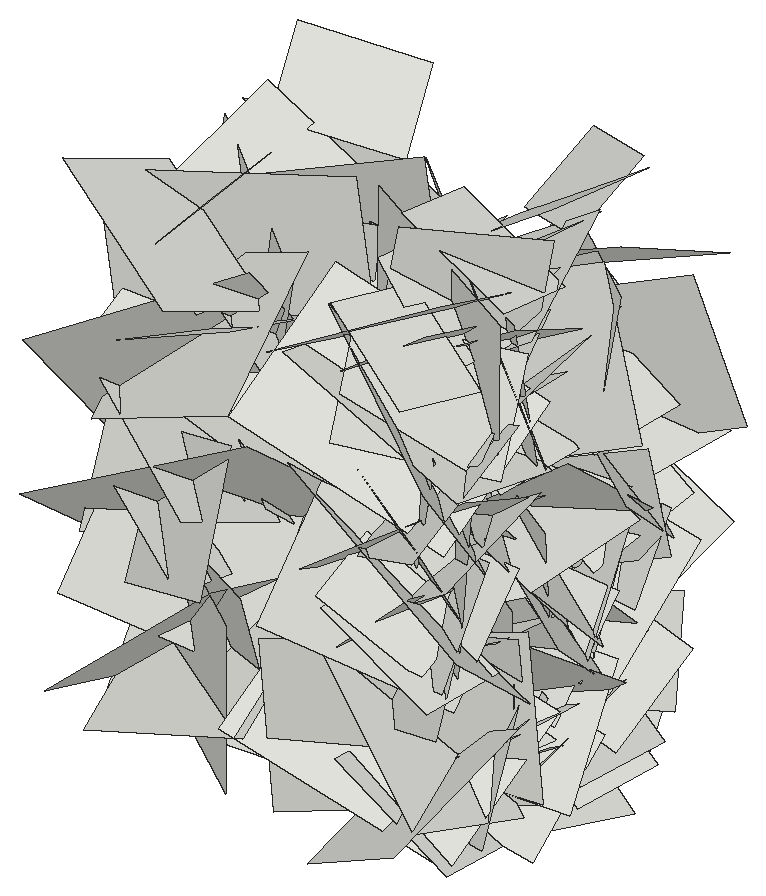
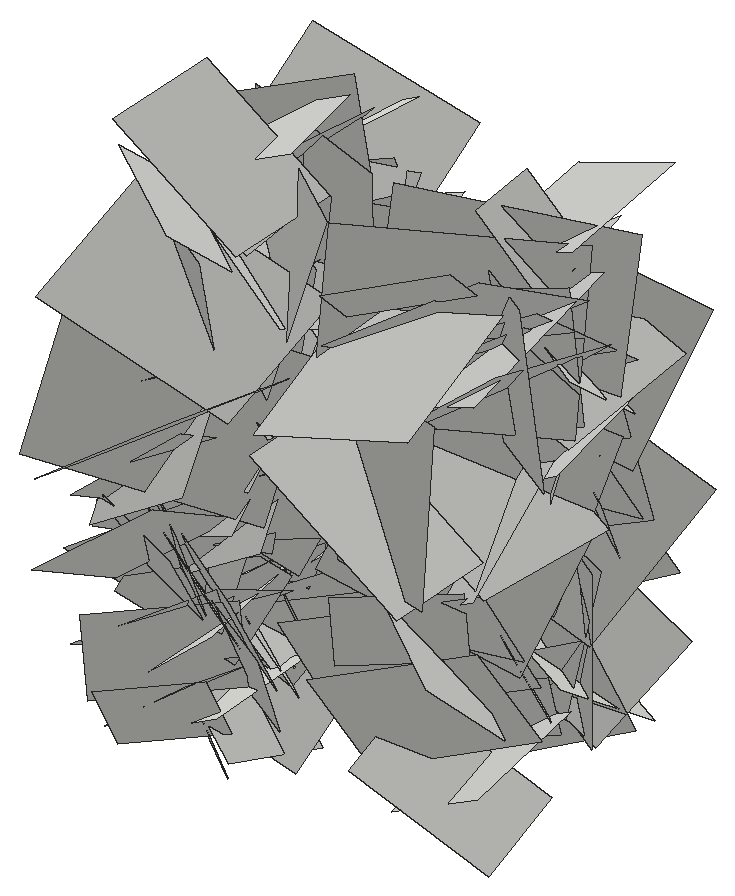
# SketchUp Ruby script. Lengths in inches.
U = 1.inch
M = Sketchup.active_model
def pt(a) = Geom::Point3d.new(a.map { |v| v * U })
def face(e, loops, mat)
  f = e.add_face(loops[0].map { |a| pt(a) })
  loops[1..].each { |l| e.add_face(l.map { |a| pt(a) }).erase! }
  f.material = f.back_material = mat if mat
  f
end
# faces: each face lists its corners as indices into pts; further lists are holes
def faces(e, pts, list, mat = nil) = list.each { |f| face(e, (f[0].is_a?(Array) ? f : [f]).map { |l| l.map { |i| pts[i] } }, mat) }
# xy, xz, yz: faces in a plane at the given z, y or x. An outline is a flat list of corners, or four numbers for a rectangle; further outlines are holes
def ring(l) = l.size == 4 ? [[l[0], l[1]], [l[2], l[1]], [l[2], l[3]], [l[0], l[3]]] : l.each_slice(2).to_a
def flat(e, list, mat, &to3) = list.each { |f| face(e, (f[0].is_a?(Array) ? f : [f]).map { |l| ring(l).map { |u, v| to3.(u, v) } }, mat) }
def xy(e, z, list, mat = nil) = flat(e, list, mat) { |x, y| [x, y, z] }
def xz(e, y, list, mat = nil) = flat(e, list, mat) { |x, z| [x, y, z] }
def yz(e, x, list, mat = nil) = flat(e, list, mat) { |y, z| [x, y, z] }
def lines(e, pts, list) = list.each { |a, b| e.add_line(pt(pts[a]), pt(pts[b])) }
# prism: a flat outline (further loops are holes) pulled along v
def prism(e, loops, v, mat = nil)
  f = face(e, loops, mat); d = Geom::Vector3d.new(v.map { |x| x * U })
  f.pushpull(f.normal.samedirection?(d) ? d.length : -d.length)
end
def box(e, o, s, mat = nil) = prism(e, [[o, [o[0] + s[0], o[1], o[2]], [o[0] + s[0], o[1] + s[1], o[2]], [o[0], o[1] + s[1], o[2]]]], [0, 0, s[2]], mat)
def at(x, y, z, deg = 0) = Geom::Transformation.translation(pt([x, y, z])) * Geom::Transformation.rotation(ORIGIN, Z_AXIS, deg.degrees)
def axes(o, x, y, z) = Geom::Transformation.new([*x, 0, *y, 0, *z, 0, *pt(o).to_a, 1])
def part(name) = M.definitions.add(name)
# library, detail: a bought-in or finely detailed component or shape, given as its bounding box
def library(name, o, s) = part(name).tap { |d| box(d.entities, o, s) }
def detail(e, o, s) = box(e.add_group.entities, o, s)
def put(e, d, t, mat = nil) = e.add_instance(d, t).tap { |i| i.material = mat if mat }
def group(e, t, mat = nil) = e.add_group.tap { |g| g.transformation = t; g.material = mat if mat }.entities
root = M.entities
c1 = part("Component\#6")
p = [[0.01,0,0],[0,3.24,4.54],[4.32,3.24,4.54],[4.33,0,0]]
faces(c1.entities,p,[[0,1,2,3]])
put(root,c1,axes([18.5,139.71,39.61],[-0.08624,0.67106,-0.00672],[0.16105,0.01183,-0.6586],[-0.69289,-0.08077,-0.15225]))
put(root,c1,axes([14.53,143.41,32.67],[-0.00295,0.89075,-0.72818],[-0.15415,-0.72261,-0.88339],[1.20976,-0.08991,-0.11434]))
put(root,c1,axes([14.53,146.5,19.86],[0.14062,-0.87102,0.18651],[0.03259,0.19294,0.87915],[0.94365,0.12313,-0.05815]))
put(root,c1,axes([14.53,145.05,38.54],[-0.26561,0.06521,-1.32838],[-0.06869,-1.35074,-0.05408],[1.4081,-0.05359,-0.25321]))
put(root,c1,axes([14.53,142.58,23.75],[0.11698,0.88265,-0.34817],[-0.00423,-0.35009,-0.88876],[1.00576,-0.10414,0.03675]))
put(root,c1,axes([14.53,141.41,21.99],[0.04242,-1.10503,0.33762],[-0.18816,0.32793,1.09436],[1.21025,0.08972,0.15831]))
put(root,c1,axes([18.5,145.49,24.46],[0.14807,-0.32942,-0.64401],[-0.00647,-0.65643,0.33444],[-0.76675,-0.05808,-0.12719]))
put(root,c1,axes([14.53,138.75,33.42],[0.07987,0.93748,-0.3836],[-0.04246,-0.3816,-0.94046],[1.07286,-0.0849,-0.00867]))
put(root,c1,axes([18.5,142.8,24.59],[0.06246,-0.31977,0.5346],[-0.03506,0.53462,0.32343],[-0.65938,-0.05871,0.03344]))
put(root,c1,axes([18.5,142.28,27.34],[0.09885,-0.42767,0.49172],[-0.03253,0.4933,0.43487],[-0.69002,-0.08452,0.04994]))
put(root,c1,axes([14.53,139.49,21.74],[0.04906,0.46783,0.90513],[0.0041,0.90598,-0.46846],[1.08001,-0.02469,-0.03934]))
put(root,c1,axes([18.5,149.12,29.1],[0.10824,-0.19319,-0.65872],[0.02698,-0.66445,0.19881],[-0.72715,-0.05341,-0.09068]))
put(root,c1,axes([14.53,145.04,25.97],[-0.0145,-0.85349,0.83598],[-0.13626,0.83223,0.84756],[1.25903,0.08024,0.10136]))
put(root,c1,axes([18.5,141.05,35.76],[0.06877,-0.60814,0.14272],[0.00885,0.14432,0.61116],[-0.66208,-0.06124,0.02299]))
put(root,c1,axes([18.5,149.56,39.6],[0.17317,-0.50739,-0.45031],[-0.03865,-0.46908,0.51531],[-0.71806,-0.09712,-0.13634]))
put(root,c1,axes([18.5,140.39,26.94],[0.03872,-0.62994,0.14227],[0.11345,0.14643,0.62088],[-0.67508,-0.01152,0.1125]))
put(root,c1,axes([18.5,144.97,35.07],[0.07722,-0.5315,-0.34657],[0.05738,-0.34237,0.53643],[-0.67013,-0.09056,0.006]))
put(root,c1,axes([14.53,139.67,30.68],[-0.09112,-0.77438,0.96294],[-0.03313,0.96632,0.77431],[1.3094,-0.02944,0.0866]))
put(root,c1,axes([14.53,138.43,27.8],[0.10648,0.28124,1.16655],[-0.16097,1.1642,-0.2676],[1.26174,0.12479,-0.13259]))
put(root,c1,axes([14.53,140.69,35.43],[0.02714,1.22478,0.26938],[-0.1382,0.27058,-1.21783],[1.3221,0.00314,-0.13283]))
put(root,c1,axes([14.53,137.65,40.3125],[0.15365,0.92766,-0.3555],[0.07441,-0.36793,-0.93147],[1.05042,-0.10963,0.11798]))
put(root,c1,axes([14.53,149.09,36.34],[-0.1737,0.35213,-1.24285],[0.08,-1.24806,-0.36356],[1.36694,0.11779,-0.13666]))
put(root,c1,axes([14.53,146.73,29.36],[-0.09029,-1.26195,0.03468],[0.03892,0.03227,1.26436],[1.33761,-0.08612,-0.03444]))
put(root,c1,axes([14.53,141.99,33.2],[0.15631,-0.03731,1.01998],[0.08418,1.02787,0.02612],[1.07863,-0.07482,-0.14985]))
put(root,c1,axes([14.53,141.2,30.22],[0.14348,-0.5033,-0.91823],[0.06175,-0.92081,0.51331],[1.10823,0.11647,0.09028]))
put(root,c1,axes([14.53,143.42,27.33],[0.08667,-0.86973,1.01008],[-0.23887,0.9884,0.86929],[1.39256,0.22367,0.08625]))
put(root,c1,axes([14.53,142.6875,32.73],[-0.11413,-1.14483,0.29443],[0.2702,0.26621,1.12831],[1.22353,-0.16558,-0.2217]))
put(root,c1,axes([14.53,143.97,23.32],[0.18437,0.48358,0.83906],[0.16998,0.82633,-0.50949],[1.01237,-0.22682,-0.06726]))
put(root,c1,axes([14.53,144,25.2],[0.04504,0.58566,0.95802],[0.11757,0.95183,-0.5868],[1.18441,-0.11675,0.02182]))
put(root,c1,axes([14.53,150.86,30.47],[0.14962,-1.13409,-0.09371],[-0.03493,-0.09847,1.14197],[1.20573,0.13788,0.04471]))
put(root,c1,axes([14.53,141.59,27.99],[-0.06396,0.08339,-1.32201],[-0.02487,-1.32324,-0.0824],[1.4039,-0.01964,-0.06169]))
put(root,c1,axes([14.53,145.76,27.48],[0.11303,-0.66031,-0.96553],[-0.02355,-0.9705,0.66125],[1.23968,0.04176,0.1006]))
put(root,c1,axes([14.53,149.48,27.53],[0.05839,-0.93868,-0.8352],[-0.07486,-0.83699,0.93604],[1.32974,-0.0059,0.08937]))
put(root,c1,axes([14.53,141.72,37.36],[0.19445,0.97106,0.50245],[-0.00165,0.50971,-0.98451],[1.15895,-0.1622,-0.0857]))
put(root,c1,axes([14.53,141.71,25.57],[-0.24627,-1.07768,0.84944],[0.21085,0.82598,1.10232],[1.43917,-0.30542,-0.01615]))
put(root,c1,axes([14.53,141.15,27.9],[0.10356,0.25866,-1.08582],[0.18317,-1.08033,-0.24181],[1.16891,0.14638,0.13409]))
put(root,c1,axes([14.53,145.83,38.68],[-0.04371,1.09164,-0.51046],[0.28885,-0.48908,-1.06793],[1.24431,0.15188,0.22998]))
put(root,c1,axes([14.53,140.25,33.3],[-0.10371,-0.10781,1.29757],[0.22808,1.282,0.12274],[1.36119,-0.22303,0.07829]))
put(root,c1,axes([14.53,139.39,34.34],[0.15089,0.92592,0.71699],[0.08883,0.71236,-0.93659],[1.23815,-0.16395,-0.02018]))
put(root,c1,axes([14.53,142.42,32.89],[0.18672,-0.42722,1.28431],[-0.1337,1.28432,0.44452],[1.42847,0.17605,-0.12627]))
put(root,c1,axes([14.53,142.63,35.02],[0.11092,-0.98462,-0.77371],[0.1183,-0.76598,0.98988],[1.32209,0.15114,-0.02366]))
put(root,c1,axes([14.53,137.42,26.21],[0.14568,0.69276,1.17725],[0.03045,1.18146,-0.69859],[1.44759,-0.09457,-0.10377]))
put(root,c1,axes([14.53,143.09,24.72],[0.05768,-1.1082,-0.74759],[0.23067,-0.73089,1.09928],[1.3981,0.16631,-0.15052]))
put(root,c1,axes([14.53,141,38.04],[0.14868,1.2474,-0.57055],[0.09146,-0.58042,-1.24775],[1.45112,-0.09122,0.1371]))
put(root,c1,axes([28.31,141,38.04],[-0.14868,1.2474,-0.57055],[-0.09146,-0.58042,-1.24775],[-1.45112,-0.09122,0.1371]))
put(root,c1,axes([28.31,143.09,24.72],[-0.05768,-1.1082,-0.74759],[-0.23067,-0.73089,1.09928],[-1.3981,0.16631,-0.15052]))
put(root,c1,axes([28.31,137.42,26.21],[-0.14568,0.69276,1.17725],[-0.03045,1.18146,-0.69859],[-1.44759,-0.09457,-0.10377]))
put(root,c1,axes([28.31,142.63,35.02],[-0.11092,-0.98462,-0.77371],[-0.1183,-0.76598,0.98988],[-1.32209,0.15114,-0.02366]))
put(root,c1,axes([28.31,142.42,32.89],[-0.18672,-0.42722,1.28431],[0.1337,1.28432,0.44452],[-1.42847,0.17605,-0.12627]))
put(root,c1,axes([28.31,139.39,34.34],[-0.15089,0.92592,0.71699],[-0.08883,0.71236,-0.93659],[-1.23815,-0.16395,-0.02018]))
put(root,c1,axes([28.31,140.25,33.3],[0.10371,-0.10781,1.29757],[-0.22808,1.282,0.12274],[-1.36119,-0.22303,0.07829]))
put(root,c1,axes([28.31,145.83,38.68],[0.04371,1.09164,-0.51046],[-0.28885,-0.48908,-1.06793],[-1.24431,0.15188,0.22998]))
put(root,c1,axes([28.31,141.15,27.9],[-0.10356,0.25866,-1.08582],[-0.18317,-1.08033,-0.24181],[-1.16891,0.14638,0.13409]))
put(root,c1,axes([28.31,141.71,25.57],[0.24627,-1.07768,0.84944],[-0.21085,0.82598,1.10232],[-1.43917,-0.30542,-0.01615]))
put(root,c1,axes([28.31,141.72,37.36],[-0.19445,0.97106,0.50245],[0.00165,0.50971,-0.98451],[-1.15895,-0.1622,-0.0857]))
put(root,c1,axes([28.31,149.48,27.53],[-0.05839,-0.93868,-0.8352],[0.07486,-0.83699,0.93604],[-1.32974,-0.0059,0.08937]))
put(root,c1,axes([28.31,145.76,27.48],[-0.11303,-0.66031,-0.96553],[0.02355,-0.9705,0.66125],[-1.23968,0.04176,0.1006]))
put(root,c1,axes([28.31,141.59,27.99],[0.06396,0.08339,-1.32201],[0.02487,-1.32324,-0.0824],[-1.4039,-0.01964,-0.06169]))
put(root,c1,axes([28.31,150.86,30.47],[-0.14962,-1.13409,-0.09371],[0.03493,-0.09847,1.14197],[-1.20573,0.13788,0.04471]))
put(root,c1,axes([28.31,144,25.2],[-0.04504,0.58566,0.95802],[-0.11757,0.95183,-0.5868],[-1.18441,-0.11675,0.02182]))
put(root,c1,axes([28.31,143.97,23.32],[-0.18437,0.48358,0.83906],[-0.16998,0.82633,-0.50949],[-1.01237,-0.22682,-0.06726]))
put(root,c1,axes([28.31,142.6875,32.73],[0.11413,-1.14483,0.29443],[-0.2702,0.26621,1.12831],[-1.22353,-0.16558,-0.2217]))
put(root,c1,axes([28.31,143.42,27.33],[-0.08667,-0.86973,1.01008],[0.23887,0.9884,0.86929],[-1.39256,0.22367,0.08625]))
put(root,c1,axes([28.31,141.2,30.22],[-0.14348,-0.5033,-0.91823],[-0.06175,-0.92081,0.51331],[-1.10823,0.11647,0.09028]))
put(root,c1,axes([28.31,141.99,33.2],[-0.15631,-0.03731,1.01998],[-0.08418,1.02787,0.02612],[-1.07863,-0.07482,-0.14985]))
put(root,c1,axes([28.31,146.73,29.36],[0.09029,-1.26195,0.03468],[-0.03892,0.03227,1.26436],[-1.33761,-0.08612,-0.03444]))
put(root,c1,axes([28.31,149.09,36.34],[0.1737,0.35213,-1.24285],[-0.08,-1.24806,-0.36356],[-1.36694,0.11779,-0.13666]))
put(root,c1,axes([28.31,137.65,40.3125],[-0.15365,0.92766,-0.3555],[-0.07441,-0.36793,-0.93147],[-1.05042,-0.10963,0.11798]))
put(root,c1,axes([28.31,140.69,35.43],[-0.02714,1.22478,0.26938],[0.1382,0.27058,-1.21783],[-1.3221,0.00314,-0.13283]))
put(root,c1,axes([28.31,138.43,27.8],[-0.10648,0.28124,1.16655],[0.16097,1.1642,-0.2676],[-1.26174,0.12479,-0.13259]))
put(root,c1,axes([28.31,139.67,30.68],[0.09112,-0.77438,0.96294],[0.03313,0.96632,0.77431],[-1.3094,-0.02944,0.0866]))
put(root,c1,axes([24.34,144.97,35.07],[-0.07722,-0.5315,-0.34657],[-0.05738,-0.34237,0.53643],[0.67013,-0.09056,0.006]))
put(root,c1,axes([24.34,140.39,26.94],[-0.03872,-0.62994,0.14227],[-0.11345,0.14643,0.62088],[0.67508,-0.01152,0.1125]))
put(root,c1,axes([24.34,149.56,39.6],[-0.17317,-0.50739,-0.45031],[0.03865,-0.46908,0.51531],[0.71806,-0.09712,-0.13634]))
put(root,c1,axes([24.34,141.05,35.76],[-0.06877,-0.60814,0.14272],[-0.00885,0.14432,0.61116],[0.66208,-0.06124,0.02299]))
put(root,c1,axes([28.31,145.04,25.97],[0.0145,-0.85349,0.83598],[0.13626,0.83223,0.84756],[-1.25903,0.08024,0.10136]))
put(root,c1,axes([24.34,149.12,29.1],[-0.10824,-0.19319,-0.65872],[-0.02698,-0.66445,0.19881],[0.72715,-0.05341,-0.09068]))
put(root,c1,axes([28.31,139.49,21.74],[-0.04906,0.46783,0.90513],[-0.0041,0.90598,-0.46846],[-1.08001,-0.02469,-0.03934]))
put(root,c1,axes([24.34,142.28,27.34],[-0.09885,-0.42767,0.49172],[0.03253,0.4933,0.43487],[0.69002,-0.08452,0.04994]))
put(root,c1,axes([24.34,142.8,24.59],[-0.06246,-0.31977,0.5346],[0.03506,0.53462,0.32343],[0.65938,-0.05871,0.03344]))
put(root,c1,axes([28.31,138.75,33.42],[-0.07987,0.93748,-0.3836],[0.04246,-0.3816,-0.94046],[-1.07286,-0.0849,-0.00867]))
put(root,c1,axes([24.34,145.49,24.46],[-0.14807,-0.32942,-0.64401],[0.00647,-0.65643,0.33444],[0.76675,-0.05808,-0.12719]))
put(root,c1,axes([28.31,141.41,21.99],[-0.04242,-1.10503,0.33762],[0.18816,0.32793,1.09436],[-1.21025,0.08972,0.15831]))
put(root,c1,axes([28.31,142.58,23.75],[-0.11698,0.88265,-0.34817],[0.00423,-0.35009,-0.88876],[-1.00576,-0.10414,0.03675]))
put(root,c1,axes([28.31,145.05,38.54],[0.26561,0.06521,-1.32838],[0.06869,-1.35074,-0.05408],[-1.4081,-0.05359,-0.25321]))
put(root,c1,axes([28.31,146.5,19.86],[-0.14062,-0.87102,0.18651],[-0.03259,0.19294,0.87915],[-0.94365,0.12313,-0.05815]))
put(root,c1,axes([28.31,143.41,32.67],[0.00295,0.89075,-0.72818],[0.15415,-0.72261,-0.88339],[-1.20976,-0.08991,-0.11434]))
put(root,c1,axes([24.34,139.71,39.61],[0.08624,0.67106,-0.00672],[-0.16105,0.01183,-0.6586],[0.69289,-0.08077,-0.15225]))
put(root,c1,axes([28.31,144.65,25.96],[-0.15377,0.53431,0.65108],[-0.06081,0.65286,-0.54856],[-0.89071,-0.13681,-0.07495]))
put(root,c1,axes([24.34,144.73,33.27],[-0.16555,-0.76551,-0.15352],[0.02389,-0.16091,0.77946],[0.82725,-0.14855,-0.05323]))
put(root,c1,axes([24.34,146.45,21.25],[-0.00375,0.2874,0.54008],[0.0654,0.5375,-0.28562],[0.64519,-0.05282,0.03209]))
put(root,c1,axes([24.34,136.92,29.78],[0.03864,0.57092,0.32429],[-0.05823,0.3263,-0.56829],[0.69355,-0.00442,-0.06578]))
put(root,c1,axes([24.34,144.18,33.46],[-0.08879,-0.56105,-0.39599],[0.0694,-0.40364,0.55803],[0.72461,-0.03009,-0.10197]))
put(root,c1,axes([28.31,149.17,29.19],[-0.22051,-0.77582,-0.34275],[0.07369,-0.36732,0.78924],[-0.89602,0.16072,0.14925]))
put(root,c1,axes([24.34,141.16,33.73],[0.01034,-0.20439,-0.70125],[-0.11317,-0.69418,0.20085],[0.76594,-0.09981,0.03914]))
put(root,c1,axes([24.34,145.72,37.21],[0.0202,-0.65006,0.07365],[-0.02062,0.07308,0.65011],[0.69316,0.02112,0.01719]))
put(root,c1,axes([24.34,146.3,23.53],[-0.0913,-0.50535,0.50896],[0.05568,0.5068,0.51209],[0.75823,-0.09807,0.02368]))
put(root,c1,axes([24.34,145.7,22.51],[-0.08358,0.19729,0.79599],[-0.0899,0.79341,-0.20506],[0.86462,0.10156,0.05562]))
put(root,c1,axes([28.31,145.12,23.07],[0.0526,-0.82286,-0.58821],[-0.0059,-0.58914,0.82367],[-1.07215,-0.03713,-0.03339]))
put(root,c1,axes([24.34,147.44,21.48],[0.11936,-0.32986,-0.48912],[-0.02265,-0.49991,0.33221],[0.62494,0.04489,0.10546]))
put(root,c1,axes([28.31,137.68,27.62],[-0.00267,0.49736,0.77514],[-0.05686,0.77375,-0.49665],[-0.97459,-0.04651,0.02685]))
put(root,c1,axes([28.31,136.3,32.46],[0.17238,0.91042,0.71253],[0.07022,0.71102,-0.92361],[-1.22345,0.16908,0.04738]))
put(root,c1,axes([24.34,137.77,24.11],[-0.1419,0.78136,-0.16109],[0.04598,-0.15597,-0.79258],[0.84441,0.13979,0.01609]))
put(root,c1,axes([24.34,143.53,22.21],[-0.15224,-0.84766,-0.36991],[-0.10957,-0.35729,0.85887],[0.97421,-0.17265,0.03879]))
put(root,c1,axes([28.31,135.48,23.28],[0.21581,1.04519,0.5846],[0.09636,0.57779,-1.06467],[-1.26577,0.22219,0.01862]))
put(root,c1,axes([24.34,145.6,27.28],[0.00806,0.29423,-0.56577],[0.12293,-0.55701,-0.28812],[0.6647,0.09945,0.06014]))
put(root,c1,axes([28.31,141.63,23.18],[0.01995,1.00092,0.30572],[0.13829,0.30114,-0.99396],[-1.10071,0.05598,-0.11933]))
put(root,c1,axes([28.31,145.42,24.52],[0.2647,-0.88765,0.75819],[0.01358,0.77738,0.90589],[-1.23735,-0.18136,0.17214]))
put(root,c1,axes([24.34,144.6,22.65],[-0.17478,-0.82558,-0.09028],[0.09417,-0.10904,0.83495],[0.87528,-0.15312,-0.10786]))
put(root,c1,axes([28.31,142.67,41.25],[0.05619,0.9574,-0.08237],[-0.00834,-0.08206,-0.95886],[-1.01856,0.05349,0.00331]))
put(root,c1,axes([28.31,148.52,32.35],[-0.08011,-0.79067,-0.06214],[-0.07476,-0.05548,0.79163],[-0.83736,0.0806,-0.06473]))
put(root,c1,axes([24.34,140.84,40.56],[-0.05261,0.712,-0.12967],[0.10362,-0.12219,-0.70833],[0.7601,0.06594,0.08758]))
put(root,c1,axes([24.34,143.38,25.93],[-0.00088,-0.66729,0.07011],[0.1194,0.06898,0.65784],[0.70113,-0.01259,-0.11194]))
put(root,c1,axes([24.34,144.05,31.85],[-0.11078,0.17753,-0.74918],[0.12323,-0.74375,-0.19246],[0.80677,0.13798,-0.07348]))
put(root,c1,axes([28.31,138.53,29.67],[-0.03677,-0.4198,0.69058],[-0.10131,0.68849,0.41374],[-0.85065,-0.06385,-0.07912]))
put(root,c1,axes([28.31,150.98,27.43],[-0.11329,-0.77541,-0.3635],[0.07754,-0.37325,0.77469],[-0.90445,0.06513,0.11195]))
put(root,c1,axes([28.31,149.13,24.11],[0.03147,-0.85153,-0.39996],[0.02133,-0.3995,0.85202],[-0.997,-0.03542,0.00561]))
put(root,c1,axes([28.31,144.71,33.13],[0.16995,0.04512,1.05289],[0.00982,1.0649,-0.04705],[-1.11704,0.01623,0.15977]))
put(root,c1,axes([24.34,143.64,28.51],[0.01569,-0.00258,-0.72773],[0.02057,-0.72762,0.00297],[0.77112,0.01947,0.01473]))
put(root,c1,axes([28.31,137.85,30.84],[0.06669,0.91948,0.38333],[0.06841,0.37952,-0.92095],[-1.05374,0.08283,-0.03553]))
put(root,c1,axes([28.31,147.08,31.53],[0.0186,0.21399,-0.90436],[0.04027,-0.90393,-0.21315],[-0.98427,-0.03294,-0.02581]))
put(root,c1,axes([24.34,144.98,23.12],[0.11015,0.70988,0.06167],[-0.04855,0.06885,-0.71532],[0.75374,-0.09931,-0.05509]))
put(root,c1,axes([24.34,140.76,35.5625],[0.0095,0.80566,-0.00603],[-0.04784,-0.00552,-0.80445],[0.85268,-0.00929,-0.04507]))
put(root,c1,axes([24.34,146.7,34.04],[-0.22474,0.77203,-0.6543],[-0.03576,-0.67353,-0.78378],[1.07212,0.13937,-0.1633]))
put(root,c1,axes([28.31,141.61,27.46],[0.15544,0.8369,-0.58263],[0.03072,-0.5918,-0.84279],[-1.08048,0.10358,-0.10778]))
put(root,c1,axes([28.31,145.6875,25.3],[0.21495,-0.77208,-0.77151],[0.06755,-0.77499,0.79232],[-1.15499,-0.18901,-0.09724]))
put(root,c1,axes([28.31,147.86,21.63],[0.08807,-1.00346,0.13322],[0.11481,0.14172,0.99989],[-1.06685,-0.06759,0.1186]))
put(root,c1,axes([24.34,139.84,37.375],[0.13047,0.02824,0.77],[-0.11824,0.77221,-0.01049],[0.80815,0.10842,-0.12584]))
put(root,c1,axes([28.31,144.76,23.61],[-0.10873,-0.7568,0.02149],[0.01122,0.02025,0.76368],[-0.80245,0.10283,0.00777]))
put(root,c1,axes([24.34,149.44,28.46],[-0.01637,-0.35652,-0.61871],[0.18604,-0.60176,0.34238],[0.7337,0.14463,-0.10062]))
put(root,c1,axes([24.34,137.14,29.31],[0.00249,0.75761,-0.01469],[0.08098,-0.01485,-0.75375],[0.79913,-0.00085,0.07643]))
put(root,c1,axes([24.34,137.53,34.5],[-0.08019,0.3809,0.76753],[0.04804,0.77121,-0.37826],[0.90698,-0.00717,0.08789]))
put(root,c1,axes([28.31,139.47,36.72],[-0.15825,-0.66033,0.08813],[-0.02764,0.09604,0.67542],[-0.70562,0.14433,-0.04622]))
